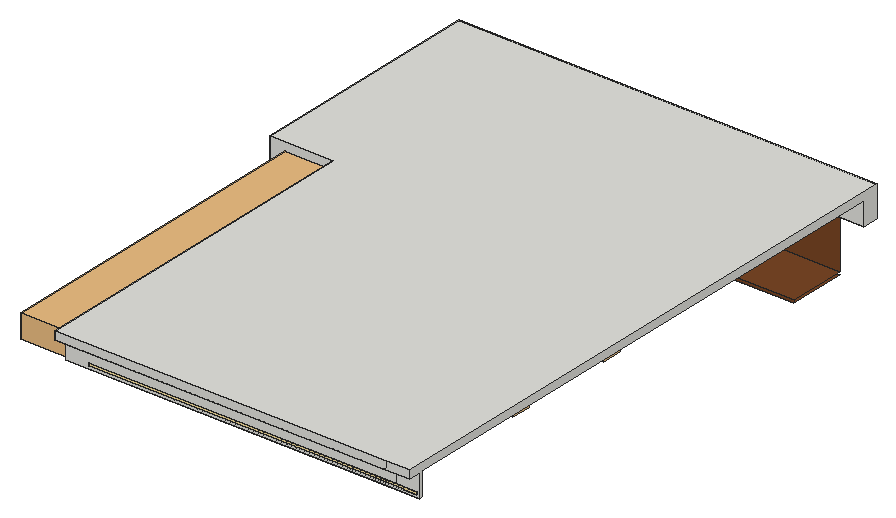
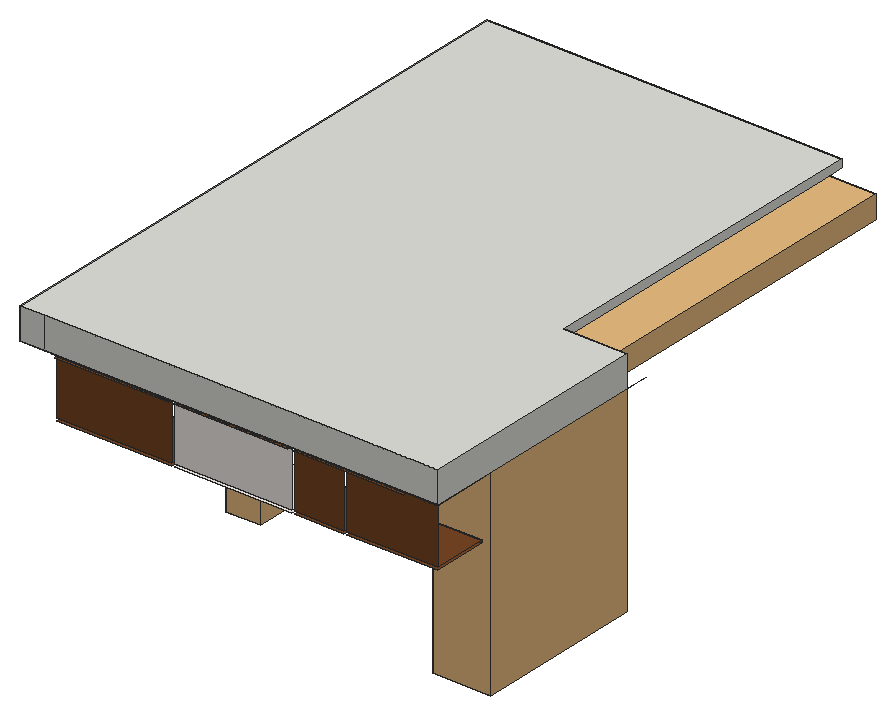
# SketchUp Ruby script. Lengths in inches.
U = 1.inch
M = Sketchup.active_model
def pt(a) = Geom::Point3d.new(a.map { |v| v * U })
def face(e, loops, mat)
  f = e.add_face(loops[0].map { |a| pt(a) })
  loops[1..].each { |l| e.add_face(l.map { |a| pt(a) }).erase! }
  f.material = f.back_material = mat if mat
  f
end
# faces: each face lists its corners as indices into pts; further lists are holes
def faces(e, pts, list, mat = nil) = list.each { |f| face(e, (f[0].is_a?(Array) ? f : [f]).map { |l| l.map { |i| pts[i] } }, mat) }
# xy, xz, yz: faces in a plane at the given z, y or x. An outline is a flat list of corners, or four numbers for a rectangle; further outlines are holes
def ring(l) = l.size == 4 ? [[l[0], l[1]], [l[2], l[1]], [l[2], l[3]], [l[0], l[3]]] : l.each_slice(2).to_a
def flat(e, list, mat, &to3) = list.each { |f| face(e, (f[0].is_a?(Array) ? f : [f]).map { |l| ring(l).map { |u, v| to3.(u, v) } }, mat) }
def xy(e, z, list, mat = nil) = flat(e, list, mat) { |x, y| [x, y, z] }
def xz(e, y, list, mat = nil) = flat(e, list, mat) { |x, z| [x, y, z] }
def yz(e, x, list, mat = nil) = flat(e, list, mat) { |y, z| [x, y, z] }
def lines(e, pts, list) = list.each { |a, b| e.add_line(pt(pts[a]), pt(pts[b])) }
# prism: a flat outline (further loops are holes) pulled along v
def prism(e, loops, v, mat = nil)
  f = face(e, loops, mat); d = Geom::Vector3d.new(v.map { |x| x * U })
  f.pushpull(f.normal.samedirection?(d) ? d.length : -d.length)
end
def box(e, o, s, mat = nil) = prism(e, [[o, [o[0] + s[0], o[1], o[2]], [o[0] + s[0], o[1] + s[1], o[2]], [o[0], o[1] + s[1], o[2]]]], [0, 0, s[2]], mat)
def at(x, y, z, deg = 0) = Geom::Transformation.translation(pt([x, y, z])) * Geom::Transformation.rotation(ORIGIN, Z_AXIS, deg.degrees)
def axes(o, x, y, z) = Geom::Transformation.new([*x, 0, *y, 0, *z, 0, *pt(o).to_a, 1])
def part(name) = M.definitions.add(name)
# library, detail: a bought-in or finely detailed component or shape, given as its bounding box
def library(name, o, s) = part(name).tap { |d| box(d.entities, o, s) }
def detail(e, o, s) = box(e.add_group.entities, o, s)
def put(e, d, t, mat = nil) = e.add_instance(d, t).tap { |i| i.material = mat if mat }
def group(e, t, mat = nil) = e.add_group.tap { |g| g.transformation = t; g.material = mat if mat }.entities
root = M.entities
M.materials.add("0001 AP 9436 AIR BREEZE").color = [243, 237, 232]
M.materials.add("False ceiling Light").color = [250, 225, 158]
M.materials.add("[Color_A11]").color = [255, 247, 241]
M.materials.add("[Wood Veneer 01]3").color = [120, 70, 37]
c1 = library("Group\#11",[0,-21.9375,2],[66,21.9375,76])
c2 = library("6",[-5.88,-5.88,-12.16],[13.32,13.32,12.16])
c3 = library("5",[-2.77,-2.77,-11.46],[7.48,7.48,11.46])
c4 = library("Group\#30",[0,0,0],[191.97,141,8.83])
xy(root,90.94,[[10,209,44.5,230],[45.5,209,64.5,230]],"[Wood Veneer 01]3")
xy(root,91,[[[65.5,208,110,230],[87.65,217.5,87.85,217.5,87.89,217.51,88.04,217.54,88.08,217.56,88.13,217.57,88.21,217.61,88.26,217.64,88.3,217.66,88.34,217.69,88.41,217.75,88.45,217.78,88.51,217.86,88.54,217.89,88.6,217.97,88.625,218.01,88.67,218.1,88.69,218.15,88.7,218.19,88.71,218.24,88.73,218.28,88.74,218.33,88.74,218.38,88.75,218.43,88.75,218.57,88.74,218.62,88.74,218.67,88.73,218.72,88.71,218.76,88.7,218.81,88.69,218.85,88.67,218.9,88.625,218.99,88.6,219.03,88.54,219.11,88.51,219.14,88.45,219.22,88.41,219.25,88.34,219.31,88.3,219.34,88.26,219.36,88.21,219.39,88.13,219.43,88.08,219.44,88.04,219.46,87.89,219.49,87.85,219.5,87.65,219.5,87.61,219.49,87.46,219.46,87.42,219.44,87.37,219.43,87.29,219.39,87.24,219.36,87.2,219.34,87.16,219.31,87.09,219.25,87.05,219.22,86.99,219.14,86.96,219.11,86.9,219.03,86.875,218.99,86.83,218.9,86.81,218.85,86.8,218.81,86.79,218.76,86.77,218.72,86.76,218.67,86.76,218.62,86.75,218.57,86.75,218.43,86.76,218.38,86.76,218.33,86.77,218.28,86.79,218.24,86.8,218.19,86.81,218.15,86.83,218.1,86.875,218.01,86.9,217.97,86.96,217.89,86.99,217.86,87.05,217.78,87.09,217.75,87.16,217.69,87.2,217.66,87.24,217.64,87.29,217.61,87.37,217.57,87.42,217.56,87.46,217.54,87.61,217.51]]],"0001 AP 9436 AIR BREEZE")
xy(root,91,[[111,208,155,230]],"[Wood Veneer 01]3")
xy(root,91.5,[[87.65,217.5,87.61,217.51,87.46,217.54,87.42,217.56,87.37,217.57,87.29,217.61,87.24,217.64,87.2,217.66,87.16,217.69,87.09,217.75,87.05,217.78,86.99,217.86,86.96,217.89,86.9,217.97,86.875,218.01,86.83,218.1,86.81,218.15,86.8,218.19,86.79,218.24,86.77,218.28,86.76,218.33,86.76,218.38,86.75,218.43,86.75,218.57,86.76,218.62,86.76,218.67,86.77,218.72,86.79,218.76,86.8,218.81,86.81,218.85,86.83,218.9,86.875,218.99,86.9,219.03,86.96,219.11,86.99,219.14,87.05,219.22,87.09,219.25,87.16,219.31,87.2,219.34,87.24,219.36,87.29,219.39,87.37,219.43,87.42,219.44,87.46,219.46,87.61,219.49,87.65,219.5,87.85,219.5,87.89,219.49,88.04,219.46,88.08,219.44,88.13,219.43,88.21,219.39,88.26,219.36,88.3,219.34,88.34,219.31,88.41,219.25,88.45,219.22,88.51,219.14,88.54,219.11,88.6,219.03,88.625,218.99,88.67,218.9,88.69,218.85,88.7,218.81,88.71,218.76,88.73,218.72,88.74,218.67,88.74,218.62,88.75,218.57,88.75,218.43,88.74,218.38,88.74,218.33,88.73,218.28,88.71,218.24,88.7,218.19,88.69,218.15,88.67,218.1,88.625,218.01,88.6,217.97,88.54,217.89,88.51,217.86,88.45,217.78,88.41,217.75,88.34,217.69,88.3,217.66,88.26,217.64,88.21,217.61,88.13,217.57,88.08,217.56,88.04,217.54,87.89,217.51,87.85,217.5]],"0001 AP 9436 AIR BREEZE")
xy(root,91.94,[[10,209,44.5,230],[45.5,209,64.5,230]],"[Wood Veneer 01]3")
xy(root,92,[[65.5,208,110,230]],"0001 AP 9436 AIR BREEZE")
xy(root,92,[[111,208,155,230]],"[Wood Veneer 01]3")
xy(root,113,[[[65.5,207,110,230],[87.65,217.5,87.85,217.5,87.89,217.51,88.04,217.54,88.08,217.56,88.13,217.57,88.21,217.61,88.26,217.64,88.3,217.66,88.34,217.69,88.41,217.75,88.45,217.78,88.51,217.86,88.54,217.89,88.6,217.97,88.625,218.01,88.67,218.1,88.69,218.15,88.7,218.19,88.71,218.24,88.73,218.28,88.74,218.33,88.74,218.38,88.75,218.43,88.75,218.57,88.74,218.62,88.74,218.67,88.73,218.72,88.71,218.76,88.7,218.81,88.69,218.85,88.67,218.9,88.625,218.99,88.6,219.03,88.54,219.11,88.51,219.14,88.45,219.22,88.41,219.25,88.34,219.31,88.3,219.34,88.26,219.36,88.21,219.39,88.13,219.43,88.08,219.44,88.04,219.46,87.89,219.49,87.85,219.5,87.65,219.5,87.61,219.49,87.46,219.46,87.42,219.44,87.37,219.43,87.29,219.39,87.24,219.36,87.2,219.34,87.16,219.31,87.09,219.25,87.05,219.22,86.99,219.14,86.96,219.11,86.9,219.03,86.875,218.99,86.83,218.9,86.81,218.85,86.8,218.81,86.79,218.76,86.77,218.72,86.76,218.67,86.76,218.62,86.75,218.57,86.75,218.43,86.76,218.38,86.76,218.33,86.77,218.28,86.79,218.24,86.8,218.19,86.81,218.15,86.83,218.1,86.875,218.01,86.9,217.97,86.96,217.89,86.99,217.86,87.05,217.78,87.09,217.75,87.16,217.69,87.2,217.66,87.24,217.64,87.29,217.61,87.37,217.57,87.42,217.56,87.46,217.54,87.61,217.51]]],"0001 AP 9436 AIR BREEZE")
xy(root,113,[[10,207,10,230,44.5,230,44.5,208,45.5,208,45.5,230,64.5,230,64.5,207],[111,207,155,230],[44.5,208,44.5,230,22,230,22,231,64,231,64,230,45.5,230,45.5,208],[66,230,109.5,231],[111.5,230,155,231]],"[Wood Veneer 01]3")
xy(root,113.5,[[87.65,217.5,87.61,217.51,87.46,217.54,87.42,217.56,87.37,217.57,87.29,217.61,87.24,217.64,87.2,217.66,87.16,217.69,87.09,217.75,87.05,217.78,86.99,217.86,86.96,217.89,86.9,217.97,86.875,218.01,86.83,218.1,86.81,218.15,86.8,218.19,86.79,218.24,86.77,218.28,86.76,218.33,86.76,218.38,86.75,218.43,86.75,218.57,86.76,218.62,86.76,218.67,86.77,218.72,86.79,218.76,86.8,218.81,86.81,218.85,86.83,218.9,86.875,218.99,86.9,219.03,86.96,219.11,86.99,219.14,87.05,219.22,87.09,219.25,87.16,219.31,87.2,219.34,87.24,219.36,87.29,219.39,87.37,219.43,87.42,219.44,87.46,219.46,87.61,219.49,87.65,219.5,87.85,219.5,87.89,219.49,88.04,219.46,88.08,219.44,88.13,219.43,88.21,219.39,88.26,219.36,88.3,219.34,88.34,219.31,88.41,219.25,88.45,219.22,88.51,219.14,88.54,219.11,88.6,219.03,88.625,218.99,88.67,218.9,88.69,218.85,88.7,218.81,88.71,218.76,88.73,218.72,88.74,218.67,88.74,218.62,88.75,218.57,88.75,218.43,88.74,218.38,88.74,218.33,88.73,218.28,88.71,218.24,88.7,218.19,88.69,218.15,88.67,218.1,88.625,218.01,88.6,217.97,88.54,217.89,88.51,217.86,88.45,217.78,88.41,217.75,88.34,217.69,88.3,217.66,88.26,217.64,88.21,217.61,88.13,217.57,88.08,217.56,88.04,217.54,87.89,217.51,87.85,217.5]],"0001 AP 9436 AIR BREEZE")
xy(root,114,[[9,207,156,231]],"[Wood Veneer 01]3")
xy(root,114.17,[[33.25,13.75,33,14,33,15,168,15,168,13.75],[33,15,33,141,9,141,9,231,168,231,168,225,156,225,156,206.97,15,206.97,15,141.5,33.25,141.5,33.25,15]])
xy(root,115.17,[[42,13.75,167,14.375]])
xy(root,116.17,[[42,13.75,167,14.375]])
xy(root,123,[[33,9,33,14,33.25,13.75,168,13.75,168,9],[[33.25,15,33.25,141.5,15,141.5,15,206.97,156,206.97,156,225,168,225,168,15],[39.25,21,162,21,162,200.97,21,200.97,21,147.5,39.25,147.5]],[39.75,21.5,39.75,148,21.5,148,21.5,200.47,161.5,200.47,161.5,21.5]])
xy(root,123.25,[[[39.25,21,39.25,147.5,21,147.5,21,200.97,162,200.97,162,21],[39.75,21.5,161.5,21.5,161.5,200.47,21.5,200.47,21.5,148,39.75,148]]])
xy(root,126,[[33,9,168,9,168,231,9,231,9,141,33,141]])
xz(root,9,[[33,123,159,126],[159,123,168,126]])
xz(root,13.75,[[33.25,114.17,159,114.17,159,115.17,42,115.17,42,116.17,159,116.17,159,123,33.25,123],[159,114.17,168,114.17,168,123,159,123,159,116.17,167,116.17,167,115.17,159,115.17]])
xz(root,14.375,[[42,115.17,167,116.17]])
xz(root,15,[[33.25,114.17,159,123],[159,114.17,168,123]])
xz(root,21,[[39.25,123,159,123.25],[159,123,162,123.25]])
xz(root,21.5,[[39.75,123,159,123.25],[159,123,161.5,123.25]])
xz(root,141,[[9,114.17,33,126]])
xz(root,141.5,[[15,114.17,33.25,123]])
xz(root,147.5,[[21,123,39.25,123.25]])
xz(root,148,[[21.5,123,39.75,123.25]])
xz(root,200.47,[[21.5,123,161.5,123.25]])
xz(root,200.97,[[21,123,162,123.25]])
xz(root,206.97,[[15,114.17,156,123]])
xz(root,208,[[65.5,91,110,92]],"0001 AP 9436 AIR BREEZE")
xz(root,208,[[111,91,155,92]],"[Wood Veneer 01]3")
xz(root,209,[[10,90.94,44.5,91.94],[45.5,90.94,64.5,91.94]],"[Wood Veneer 01]3")
xz(root,217.5,[[87.65,91,87.7,91.5],[87.7,91,87.75,91.5],[87.75,91,87.8,91.5],[87.8,91,87.85,91.5],[87.65,113,87.7,113.5],
  [87.7,113,87.75,113.5],[87.75,113,87.8,113.5],[87.8,113,87.85,113.5]],"0001 AP 9436 AIR BREEZE")
xz(root,219.5,[[87.65,91,87.7,91.5],[87.7,91,87.75,91.5],[87.75,91,87.8,91.5],[87.8,91,87.85,91.5],[87.65,113,87.7,113.5],
  [87.7,113,87.75,113.5],[87.75,113,87.8,113.5],[87.8,113,87.85,113.5]],"0001 AP 9436 AIR BREEZE")
xz(root,225,[[156,114.17,159,123],[159,114.17,168,123]])
xz(root,230,[[65.5,92,110,113]],"0001 AP 9436 AIR BREEZE")
xz(root,230,[[10,91.94,44.5,113],[45.5,91.94,64.5,113],[111,92,155,113]],"[Wood Veneer 01]3")
xz(root,231,[[9,114.17,159,126],[159,114.17,168,126]])
yz(root,9,[[141,114.17,231,126]])
yz(root,15,[[141.5,114.17,206.97,123]])
yz(root,21,[[147.5,123,200.97,123.25]])
yz(root,21.5,[[148,123,200.47,123.25]])
yz(root,33,[[14,114.17,14,123,9,123,9,126,141,126,141,114.17]])
yz(root,33.25,[[15,114.17,141.5,123]])
yz(root,39.25,[[21,123,147.5,123.25]])
yz(root,39.75,[[21.5,123,148,123.25]])
yz(root,42,[[13.75,115.17,14.375,116.17]])
yz(root,86.75,[[218.43,91,218.48,91.5],[218.48,91,218.52,91.5],[218.52,91,218.57,91.5],[218.43,113,218.48,113.5],[218.48,113,218.52,113.5],
  [218.52,113,218.57,113.5]],"0001 AP 9436 AIR BREEZE")
yz(root,86.76,[[218.33,91,218.38,91.5],[218.62,91,218.67,91.5],[218.33,113,218.38,113.5],[218.62,113,218.67,113.5]],"0001 AP 9436 AIR BREEZE")
yz(root,88.74,[[218.33,91,218.38,91.5],[218.62,91,218.67,91.5],[218.33,113,218.38,113.5],[218.62,113,218.67,113.5]],"0001 AP 9436 AIR BREEZE")
yz(root,88.75,[[218.43,91,218.48,91.5],[218.48,91,218.52,91.5],[218.52,91,218.57,91.5],[218.43,113,218.48,113.5],[218.48,113,218.52,113.5],
  [218.52,113,218.57,113.5]],"0001 AP 9436 AIR BREEZE")
yz(root,156,[[206.97,114.17,225,123]])
yz(root,161.5,[[21.5,123,200.47,123.25]])
yz(root,162,[[21,123,200.97,123.25]])
yz(root,167,[[13.75,115.17,14.375,116.17]])
yz(root,168,[[13.75,114.17,15,114.17,15,123,225,123,225,114.17,231,114.17,231,126,9,126,9,123,13.75,123]])
p = [[87.46,217.54,91],[87.42,217.56,91],[87.42,217.56,91.5],[87.46,217.54,91.5],[87.56,217.52,91],[87.51,217.53,91],
  [87.51,217.53,91.5],[87.56,217.52,91.5],[87.65,217.5,91],[87.61,217.51,91],[87.61,217.51,91.5],[87.65,217.5,91.5],
  [87.89,217.51,91],[87.85,217.5,91],[87.85,217.5,91.5],[87.89,217.51,91.5],[87.99,217.53,91],[87.94,217.52,91],
  [87.94,217.52,91.5],[87.99,217.53,91.5],[88.08,217.56,91],[88.04,217.54,91],[88.04,217.54,91.5],[88.08,217.56,91.5],
  [87.29,217.61,91],[87.24,217.64,91],[87.24,217.64,91.5],[87.29,217.61,91.5],[87.2,217.66,91],[87.2,217.66,91.5],
  [87.37,217.57,91],[87.33,217.59,91],[87.33,217.59,91.5],[87.37,217.57,91.5],[88.17,217.59,91],[88.13,217.57,91],
  [88.13,217.57,91.5],[88.17,217.59,91.5],[88.26,217.64,91],[88.21,217.61,91],[88.21,217.61,91.5],[88.26,217.64,91.5],
  [88.3,217.66,91],[88.3,217.66,91.5],[87.16,217.69,91],[87.125,217.72,91],[87.125,217.72,91.5],[87.16,217.69,91.5],
  [87.09,217.75,91],[87.09,217.75,91.5],[88.375,217.72,91],[88.34,217.69,91],[88.34,217.69,91.5],[88.375,217.72,91.5],
  [88.41,217.75,91],[88.41,217.75,91.5],[87.05,217.78,91],[87.02,217.82,91],[87.02,217.82,91.5],[87.05,217.78,91.5],
  [86.99,217.86,91],[86.99,217.86,91.5],[88.48,217.82,91],[88.45,217.78,91],[88.45,217.78,91.5],[88.48,217.82,91.5],
  [88.51,217.86,91],[88.51,217.86,91.5],[86.96,217.89,91],[86.93,217.93,91],[86.93,217.93,91.5],[86.96,217.89,91.5],
  [86.9,217.97,91],[86.9,217.97,91.5],[88.57,217.93,91],[88.54,217.89,91],[88.54,217.89,91.5],[88.57,217.93,91.5],
  [88.6,217.97,91],[88.6,217.97,91.5],[86.875,218.01,91],[86.875,218.01,91.5],[86.85,218.06,91],[86.85,218.06,91.5],
  [88.65,218.06,91],[88.625,218.01,91],[88.625,218.01,91.5],[88.65,218.06,91.5],[86.83,218.1,91],[86.83,218.1,91.5],
  [86.81,218.15,91],[86.81,218.15,91.5],[86.8,218.19,91],[86.8,218.19,91.5],[88.67,218.1,91],[88.67,218.1,91.5],
  [88.7,218.19,91],[88.69,218.15,91],[88.69,218.15,91.5],[88.7,218.19,91.5],[86.79,218.24,91],[86.79,218.24,91.5],
  [86.77,218.28,91],[86.77,218.28,91.5],[88.73,218.28,91],[88.71,218.24,91],[88.71,218.24,91.5],[88.73,218.28,91.5],
  [86.76,218.33,91],[86.76,218.33,91.5],[88.74,218.33,91],[88.74,218.33,91.5],[86.76,218.38,91],[86.75,218.43,91],
  [86.75,218.43,91.5],[86.76,218.38,91.5],[88.75,218.43,91],[88.74,218.38,91],[88.74,218.38,91.5],[88.75,218.43,91.5],
  [86.75,218.57,91],[86.76,218.62,91],[86.76,218.62,91.5],[86.75,218.57,91.5],[88.74,218.62,91],[88.75,218.57,91],
  [88.75,218.57,91.5],[88.74,218.62,91.5],[86.76,218.67,91],[86.77,218.72,91],[86.77,218.72,91.5],[86.76,218.67,91.5],
  [86.79,218.76,91],[86.79,218.76,91.5],[88.71,218.76,91],[88.73,218.72,91],[88.73,218.72,91.5],[88.71,218.76,91.5],
  [88.74,218.67,91],[88.74,218.67,91.5],[86.8,218.81,91],[86.8,218.81,91.5],[86.81,218.85,91],[86.81,218.85,91.5],
  [88.69,218.85,91],[88.7,218.81,91],[88.7,218.81,91.5],[88.69,218.85,91.5],[86.83,218.9,91],[86.83,218.9,91.5],
  [86.85,218.94,91],[86.85,218.94,91.5],[86.875,218.99,91],[86.875,218.99,91.5],[88.625,218.99,91],[88.65,218.94,91],
  [88.65,218.94,91.5],[88.625,218.99,91.5],[88.67,218.9,91],[88.67,218.9,91.5],[86.9,219.03,91],[86.9,219.03,91.5],
  [86.93,219.07,91],[86.93,219.07,91.5],[88.57,219.07,91],[88.6,219.03,91],[88.6,219.03,91.5],[88.57,219.07,91.5],
  [86.96,219.11,91],[86.96,219.11,91.5],[86.99,219.14,91],[86.99,219.14,91.5],[87.02,219.18,91],[87.02,219.18,91.5],
  [88.48,219.18,91],[88.51,219.14,91],[88.51,219.14,91.5],[88.48,219.18,91.5],[88.54,219.11,91],[88.54,219.11,91.5],
  [87.05,219.22,91],[87.05,219.22,91.5],[87.09,219.25,91],[87.09,219.25,91.5],[87.125,219.28,91],[87.125,219.28,91.5],
  [88.375,219.28,91],[88.41,219.25,91],[88.41,219.25,91.5],[88.375,219.28,91.5],[88.45,219.22,91],[88.45,219.22,91.5],
  [87.16,219.31,91],[87.16,219.31,91.5],[87.2,219.34,91],[87.2,219.34,91.5],[87.24,219.36,91],[87.24,219.36,91.5],
  [88.26,219.36,91],[88.3,219.34,91],[88.3,219.34,91.5],[88.26,219.36,91.5],[88.34,219.31,91],[88.34,219.31,91.5],
  [87.29,219.39,91],[87.29,219.39,91.5],[87.33,219.41,91],[87.33,219.41,91.5],[87.37,219.43,91],[87.37,219.43,91.5],
  [87.42,219.44,91],[87.42,219.44,91.5],[87.46,219.46,91],[87.46,219.46,91.5],[88.04,219.46,91],[88.08,219.44,91],
  [88.08,219.44,91.5],[88.04,219.46,91.5],[88.13,219.43,91],[88.13,219.43,91.5],[88.17,219.41,91],[88.17,219.41,91.5],
  [88.21,219.39,91],[88.21,219.39,91.5],[87.51,219.47,91],[87.51,219.47,91.5],[87.56,219.48,91],[87.56,219.48,91.5],
  [87.61,219.49,91],[87.61,219.49,91.5],[87.65,219.5,91],[87.65,219.5,91.5],[87.85,219.5,91],[87.89,219.49,91],
  [87.89,219.49,91.5],[87.85,219.5,91.5],[87.94,219.48,91],[87.94,219.48,91.5],[87.99,219.47,91],[87.99,219.47,91.5],
  [87.46,217.54,113],[87.42,217.56,113],[87.42,217.56,113.5],[87.46,217.54,113.5],[87.56,217.52,113],[87.51,217.53,113],
  [87.51,217.53,113.5],[87.56,217.52,113.5],[87.65,217.5,113],[87.61,217.51,113],[87.61,217.51,113.5],[87.65,217.5,113.5],
  [87.89,217.51,113],[87.85,217.5,113],[87.85,217.5,113.5],[87.89,217.51,113.5],[87.99,217.53,113],[87.94,217.52,113],
  [87.94,217.52,113.5],[87.99,217.53,113.5],[88.08,217.56,113],[88.04,217.54,113],[88.04,217.54,113.5],[88.08,217.56,113.5],
  [87.29,217.61,113],[87.24,217.64,113],[87.24,217.64,113.5],[87.29,217.61,113.5],[87.2,217.66,113],[87.2,217.66,113.5],
  [87.37,217.57,113],[87.33,217.59,113],[87.33,217.59,113.5],[87.37,217.57,113.5],[88.17,217.59,113],[88.13,217.57,113],
  [88.13,217.57,113.5],[88.17,217.59,113.5],[88.26,217.64,113],[88.21,217.61,113],[88.21,217.61,113.5],[88.26,217.64,113.5],
  [88.3,217.66,113],[88.3,217.66,113.5],[87.16,217.69,113],[87.125,217.72,113],[87.125,217.72,113.5],[87.16,217.69,113.5],
  [87.09,217.75,113],[87.09,217.75,113.5],[88.375,217.72,113],[88.34,217.69,113],[88.34,217.69,113.5],[88.375,217.72,113.5],
  [88.41,217.75,113],[88.41,217.75,113.5],[87.05,217.78,113],[87.02,217.82,113],[87.02,217.82,113.5],[87.05,217.78,113.5],
  [86.99,217.86,113],[86.99,217.86,113.5],[88.48,217.82,113],[88.45,217.78,113],[88.45,217.78,113.5],[88.48,217.82,113.5],
  [88.51,217.86,113],[88.51,217.86,113.5],[86.96,217.89,113],[86.93,217.93,113],[86.93,217.93,113.5],[86.96,217.89,113.5],
  [86.9,217.97,113],[86.9,217.97,113.5],[88.57,217.93,113],[88.54,217.89,113],[88.54,217.89,113.5],[88.57,217.93,113.5],
  [88.6,217.97,113],[88.6,217.97,113.5],[86.875,218.01,113],[86.875,218.01,113.5],[86.85,218.06,113],[86.85,218.06,113.5],
  [88.65,218.06,113],[88.625,218.01,113],[88.625,218.01,113.5],[88.65,218.06,113.5],[86.83,218.1,113],[86.83,218.1,113.5],
  [86.81,218.15,113],[86.81,218.15,113.5],[86.8,218.19,113],[86.8,218.19,113.5],[88.67,218.1,113],[88.67,218.1,113.5],
  [88.7,218.19,113],[88.69,218.15,113],[88.69,218.15,113.5],[88.7,218.19,113.5],[86.79,218.24,113],[86.79,218.24,113.5],
  [86.77,218.28,113],[86.77,218.28,113.5],[88.73,218.28,113],[88.71,218.24,113],[88.71,218.24,113.5],[88.73,218.28,113.5],
  [86.76,218.33,113],[86.76,218.33,113.5],[88.74,218.33,113],[88.74,218.33,113.5],[86.76,218.38,113],[86.75,218.43,113],
  [86.75,218.43,113.5],[86.76,218.38,113.5],[88.75,218.43,113],[88.74,218.38,113],[88.74,218.38,113.5],[88.75,218.43,113.5],
  [86.75,218.57,113],[86.76,218.62,113],[86.76,218.62,113.5],[86.75,218.57,113.5],[88.74,218.62,113],[88.75,218.57,113],
  [88.75,218.57,113.5],[88.74,218.62,113.5],[86.76,218.67,113],[86.77,218.72,113],[86.77,218.72,113.5],[86.76,218.67,113.5],
  [86.79,218.76,113],[86.79,218.76,113.5],[88.71,218.76,113],[88.73,218.72,113],[88.73,218.72,113.5],[88.71,218.76,113.5],
  [88.74,218.67,113],[88.74,218.67,113.5],[86.8,218.81,113],[86.8,218.81,113.5],[86.81,218.85,113],[86.81,218.85,113.5],
  [88.69,218.85,113],[88.7,218.81,113],[88.7,218.81,113.5],[88.69,218.85,113.5],[86.83,218.9,113],[86.83,218.9,113.5],
  [86.85,218.94,113],[86.85,218.94,113.5],[86.875,218.99,113],[86.875,218.99,113.5],[88.625,218.99,113],[88.65,218.94,113],
  [88.65,218.94,113.5],[88.625,218.99,113.5],[88.67,218.9,113],[88.67,218.9,113.5],[86.9,219.03,113],[86.9,219.03,113.5],
  [86.93,219.07,113],[86.93,219.07,113.5],[88.57,219.07,113],[88.6,219.03,113],[88.6,219.03,113.5],[88.57,219.07,113.5],
  [86.96,219.11,113],[86.96,219.11,113.5],[86.99,219.14,113],[86.99,219.14,113.5],[87.02,219.18,113],[87.02,219.18,113.5],
  [88.48,219.18,113],[88.51,219.14,113],[88.51,219.14,113.5],[88.48,219.18,113.5],[88.54,219.11,113],[88.54,219.11,113.5],
  [87.05,219.22,113],[87.05,219.22,113.5],[87.09,219.25,113],[87.09,219.25,113.5],[87.125,219.28,113],[87.125,219.28,113.5],
  [88.375,219.28,113],[88.41,219.25,113],[88.41,219.25,113.5],[88.375,219.28,113.5],[88.45,219.22,113],[88.45,219.22,113.5],
  [87.16,219.31,113],[87.16,219.31,113.5],[87.2,219.34,113],[87.2,219.34,113.5],[87.24,219.36,113],[87.24,219.36,113.5],
  [88.26,219.36,113],[88.3,219.34,113],[88.3,219.34,113.5],[88.26,219.36,113.5],[88.34,219.31,113],[88.34,219.31,113.5],
  [87.29,219.39,113],[87.29,219.39,113.5],[87.33,219.41,113],[87.33,219.41,113.5],[87.37,219.43,113],[87.37,219.43,113.5],
  [87.42,219.44,113],[87.42,219.44,113.5],[87.46,219.46,113],[87.46,219.46,113.5],[88.04,219.46,113],[88.08,219.44,113],
  [88.08,219.44,113.5],[88.04,219.46,113.5],[88.13,219.43,113],[88.13,219.43,113.5],[88.17,219.41,113],[88.17,219.41,113.5],
  [88.21,219.39,113],[88.21,219.39,113.5],[87.51,219.47,113],[87.51,219.47,113.5],[87.56,219.48,113],[87.56,219.48,113.5],
  [87.61,219.49,113],[87.61,219.49,113.5],[87.65,219.5,113],[87.65,219.5,113.5],[87.85,219.5,113],[87.89,219.49,113],
  [87.89,219.49,113.5],[87.85,219.5,113.5],[87.94,219.48,113],[87.94,219.48,113.5],[87.99,219.47,113],[87.99,219.47,113.5],
  [33.25,13.75,123],[33,14,123],[33,14,114.17],[33.25,13.75,114.17],[9,141,114.17],[9,132,114.17],
  [24,141,114.17],[24,132,114.17]]
faces(root,p,[[0,1,2,3],[4,5,6,7],[5,0,3,6],[8,9,10,11],[9,4,7,10],[12,13,14,15],[16,17,18,19],[17,12,15,18],
  [20,21,22,23],[21,16,19,22],[24,25,26,27],[25,28,29,26],[30,31,32,33],[31,24,27,32],[1,30,33,2],[34,35,36,37],
  [35,20,23,36],[38,39,40,41],[39,34,37,40],[42,38,41,43],[44,45,46,47],[45,48,49,46],[28,44,47,29],[50,51,52,53],
  [51,42,43,52],[54,50,53,55],[56,57,58,59],[57,60,61,58],[48,56,59,49],[62,63,64,65],[63,54,55,64],[66,62,65,67],
  [68,69,70,71],[69,72,73,70],[60,68,71,61],[74,75,76,77],[75,66,67,76],[78,74,77,79],[72,80,81,73],[80,82,83,81],
  [84,85,86,87],[85,78,79,86],[82,88,89,83],[88,90,91,89],[90,92,93,91],[94,84,87,95],[96,97,98,99],[97,94,95,98],
  [92,100,101,93],[100,102,103,101],[104,105,106,107],[105,96,99,106],[102,108,109,103],[110,104,107,111],[112,113,114,115],[116,117,118,119],
  [120,121,122,123],[124,125,126,127],[128,129,130,131],[129,132,133,130],[134,135,136,137],[135,138,139,136],[132,140,141,133],[140,142,143,141],
  [144,145,146,147],[145,134,137,146],[142,148,149,143],[148,150,151,149],[150,152,153,151],[154,155,156,157],[155,158,159,156],[158,144,147,159],
  [152,160,161,153],[160,162,163,161],[164,165,166,167],[165,154,157,166],[162,168,169,163],[168,170,171,169],[170,172,173,171],[174,175,176,177],
  [175,178,179,176],[178,164,167,179],[172,180,181,173],[180,182,183,181],[182,184,185,183],[186,187,188,189],[187,190,191,188],[190,174,177,191],
  [184,192,193,185],[192,194,195,193],[194,196,197,195],[198,199,200,201],[199,202,203,200],[202,186,189,203],[196,204,205,197],[204,206,207,205],
  [206,208,209,207],[208,210,211,209],[210,212,213,211],[214,215,216,217],[215,218,219,216],[218,220,221,219],[220,222,223,221],[222,198,201,223],
  [212,224,225,213],[224,226,227,225],[226,228,229,227],[228,230,231,229],[232,233,234,235],[233,236,237,234],[236,238,239,237],[238,214,217,239],
  [240,241,242,243],[244,245,246,247],[245,240,243,246],[248,249,250,251],[249,244,247,250],[252,253,254,255],[256,257,258,259],[257,252,255,258],
  [260,261,262,263],[261,256,259,262],[264,265,266,267],[265,268,269,266],[270,271,272,273],[271,264,267,272],[241,270,273,242],[274,275,276,277],
  [275,260,263,276],[278,279,280,281],[279,274,277,280],[282,278,281,283],[284,285,286,287],[285,288,289,286],[268,284,287,269],[290,291,292,293],
  [291,282,283,292],[294,290,293,295],[296,297,298,299],[297,300,301,298],[288,296,299,289],[302,303,304,305],[303,294,295,304],[306,302,305,307],
  [308,309,310,311],[309,312,313,310],[300,308,311,301],[314,315,316,317],[315,306,307,316],[318,314,317,319],[312,320,321,313],[320,322,323,321],
  [324,325,326,327],[325,318,319,326],[322,328,329,323],[328,330,331,329],[330,332,333,331],[334,324,327,335],[336,337,338,339],[337,334,335,338],
  [332,340,341,333],[340,342,343,341],[344,345,346,347],[345,336,339,346],[342,348,349,343],[350,344,347,351],[352,353,354,355],[356,357,358,359],
  [360,361,362,363],[364,365,366,367],[368,369,370,371],[369,372,373,370],[374,375,376,377],[375,378,379,376],[372,380,381,373],[380,382,383,381],
  [384,385,386,387],[385,374,377,386],[382,388,389,383],[388,390,391,389],[390,392,393,391],[394,395,396,397],[395,398,399,396],[398,384,387,399],
  [392,400,401,393],[400,402,403,401],[404,405,406,407],[405,394,397,406],[402,408,409,403],[408,410,411,409],[410,412,413,411],[414,415,416,417],
  [415,418,419,416],[418,404,407,419],[412,420,421,413],[420,422,423,421],[422,424,425,423],[426,427,428,429],[427,430,431,428],[430,414,417,431],
  [424,432,433,425],[432,434,435,433],[434,436,437,435],[438,439,440,441],[439,442,443,440],[442,426,429,443],[436,444,445,437],[444,446,447,445],
  [446,448,449,447],[448,450,451,449],[450,452,453,451],[454,455,456,457],[455,458,459,456],[458,460,461,459],[460,462,463,461],[462,438,441,463],
  [452,464,465,453],[464,466,467,465],[466,468,469,467],[468,470,471,469],[472,473,474,475],[473,476,477,474],[476,478,479,477],[478,454,457,479]],"0001 AP 9436 AIR BREEZE")
faces(root,p,[[480,481,482,483]])
lines(root,p,[[484,485],[486,487]])
put(root,c1,axes([9,141,36],[0,0.98485,0],[-1,0,0],[0,0,1]),"[Color_A11]")
put(root,c2,at(88.53,217.72,91.34,90),"[Wood Veneer 01]3")
put(root,c2,at(88.53,217.72,113.4,90),"[Wood Veneer 01]3")
put(root,c3,at(110.47,173.03,118.35,90))
put(root,c3,at(143.97,169.03,118.35,90))
put(root,c3,at(72.97,169.03,118.35,90))
put(root,c3,at(72.97,125.7,118.35,90))
put(root,c3,at(72.97,82.36,118.35,90))
put(root,c3,at(72.97,39.03,118.35,90))
put(root,c3,at(110.47,35.03,118.35,90))
put(root,c3,at(147.97,125.7,118.35,90))
put(root,c3,at(147.97,82.36,118.35,90))
put(root,c3,at(143.97,39.03,118.35,90))
put(root,c4,at(156,15,114.17,90))
g1 = group(root,at(168,14.375,115.17,90),"False ceiling Light")
box(g1,[-0.625,1,0],[0.625,125,1])
